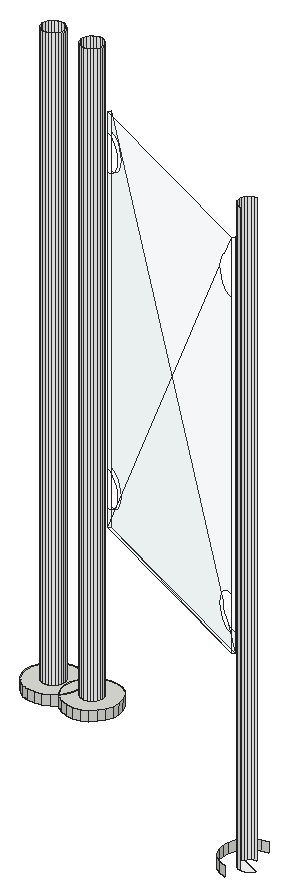
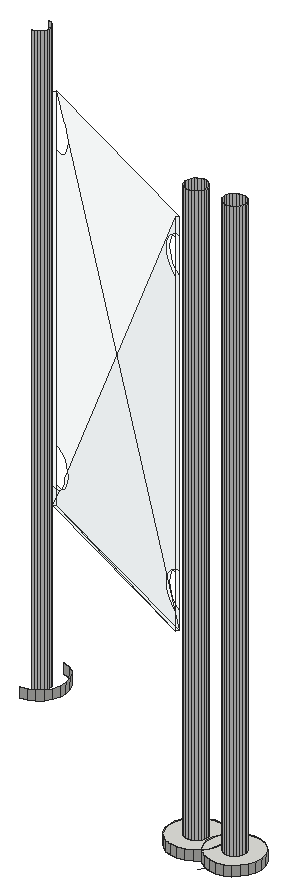
# SketchUp Ruby script. Lengths in inches.
U = 1.inch
M = Sketchup.active_model
def pt(a) = Geom::Point3d.new(a.map { |v| v * U })
def face(e, loops, mat)
  f = e.add_face(loops[0].map { |a| pt(a) })
  loops[1..].each { |l| e.add_face(l.map { |a| pt(a) }).erase! }
  f.material = f.back_material = mat if mat
  f
end
# faces: each face lists its corners as indices into pts; further lists are holes
def faces(e, pts, list, mat = nil) = list.each { |f| face(e, (f[0].is_a?(Array) ? f : [f]).map { |l| l.map { |i| pts[i] } }, mat) }
# xy, xz, yz: faces in a plane at the given z, y or x. An outline is a flat list of corners, or four numbers for a rectangle; further outlines are holes
def ring(l) = l.size == 4 ? [[l[0], l[1]], [l[2], l[1]], [l[2], l[3]], [l[0], l[3]]] : l.each_slice(2).to_a
def flat(e, list, mat, &to3) = list.each { |f| face(e, (f[0].is_a?(Array) ? f : [f]).map { |l| ring(l).map { |u, v| to3.(u, v) } }, mat) }
def xy(e, z, list, mat = nil) = flat(e, list, mat) { |x, y| [x, y, z] }
def xz(e, y, list, mat = nil) = flat(e, list, mat) { |x, z| [x, y, z] }
def yz(e, x, list, mat = nil) = flat(e, list, mat) { |y, z| [x, y, z] }
def lines(e, pts, list) = list.each { |a, b| e.add_line(pt(pts[a]), pt(pts[b])) }
# prism: a flat outline (further loops are holes) pulled along v
def prism(e, loops, v, mat = nil)
  f = face(e, loops, mat); d = Geom::Vector3d.new(v.map { |x| x * U })
  f.pushpull(f.normal.samedirection?(d) ? d.length : -d.length)
end
def box(e, o, s, mat = nil) = prism(e, [[o, [o[0] + s[0], o[1], o[2]], [o[0] + s[0], o[1] + s[1], o[2]], [o[0], o[1] + s[1], o[2]]]], [0, 0, s[2]], mat)
def at(x, y, z, deg = 0) = Geom::Transformation.translation(pt([x, y, z])) * Geom::Transformation.rotation(ORIGIN, Z_AXIS, deg.degrees)
def axes(o, x, y, z) = Geom::Transformation.new([*x, 0, *y, 0, *z, 0, *pt(o).to_a, 1])
def part(name) = M.definitions.add(name)
# library, detail: a bought-in or finely detailed component or shape, given as its bounding box
def library(name, o, s) = part(name).tap { |d| box(d.entities, o, s) }
def detail(e, o, s) = box(e.add_group.entities, o, s)
def put(e, d, t, mat = nil) = e.add_instance(d, t).tap { |i| i.material = mat if mat }
def group(e, t, mat = nil) = e.add_group.tap { |g| g.transformation = t; g.material = mat if mat }.entities
root = M.entities
M.materials.add("Glass_Safety_01").color = [204, 235, 244]
M.materials["Glass_Safety_01"].alpha = 0.1
M.materials.add("[Color_000]").color = [255, 255, 255]
xy(root,321.267,[[[557.192,657.767,557.595,657.85,557.962,658.034,558.139,658.191,558.27,658.307,558.496,658.65,558.626,659.04,558.65,659.451,558.568,659.854,558.383,660.221,558.111,660.529,557.767,660.755,557.377,660.885,556.967,660.909,556.564,660.826,556.197,660.642,555.901,660.38,555.889,660.369,555.663,660.026,555.533,659.636,555.529,659.561,555.509,659.226,555.591,658.823,555.775,658.455,555.88,658.337,556.048,658.148,556.392,657.922,556.782,657.792],[557.124,658.71,556.96,658.72,556.804,658.772,556.8,658.774,556.667,658.862,556.558,658.985,556.484,659.132,556.451,659.293,556.461,659.457,556.513,659.613,556.603,659.751,556.726,659.86,556.873,659.933,557.034,659.967,557.199,659.957,557.355,659.905,557.492,659.814,557.601,659.691,557.675,659.544,557.708,659.383,557.698,659.219,557.646,659.063,557.556,658.926,557.433,658.817,557.286,658.743]],[[554.814,657.808,555.217,657.891,555.585,658.075,555.88,658.337,555.892,658.348,556.118,658.691,556.231,659.029,556.248,659.081,556.273,659.492,556.19,659.894,556.006,660.262,555.901,660.38,555.733,660.569,555.39,660.796,555.343,660.811,555,660.925,554.589,660.95,554.186,660.867,553.819,660.683,553.511,660.41,553.285,660.067,553.155,659.677,553.131,659.266,553.214,658.864,553.398,658.496,553.671,658.189,554.014,657.962,554.404,657.833],[554.747,658.751,554.583,658.76,554.427,658.812,554.289,658.903,554.18,659.026,554.107,659.173,554.073,659.334,554.083,659.498,554.135,659.654,554.226,659.791,554.349,659.901,554.496,659.974,554.657,660.007,554.821,659.997,554.977,659.946,555.114,659.855,555.223,659.732,555.297,659.585,555.33,659.424,555.32,659.26,555.268,659.104,555.178,658.966,555.055,658.857,554.908,658.784]],[558.139,658.191,558.27,658.307,558.496,658.65,558.626,659.04,558.65,659.451,558.568,659.854,558.383,660.221,558.111,660.529,557.767,660.755,557.377,660.885,556.967,660.909,556.564,660.826,556.197,660.642,555.901,660.38,555.733,660.569,555.39,660.796,555.343,660.811,555.326,660.757,555.304,660.668,555.287,660.578,555.276,660.487,555.272,660.395,555.273,660.303,555.28,660.212,555.294,660.121,555.313,660.031,555.338,659.943,555.369,659.857,555.405,659.772,555.447,659.691,555.494,659.612,555.529,659.561,555.546,659.536,555.603,659.464,555.664,659.396,555.73,659.332,555.8,659.273,555.874,659.218,555.951,659.168,556.031,659.123,556.231,659.029,556.389,658.953,556.8,658.774,556.667,658.862,556.558,658.985,556.484,659.132,556.451,659.293,556.461,659.457,556.513,659.613,556.603,659.751,556.726,659.86,556.873,659.933,557.034,659.967,557.199,659.957,557.355,659.905,557.492,659.814,557.601,659.691,557.675,659.544,557.708,659.383,557.698,659.219,557.646,659.063,557.556,658.926,557.433,658.817,557.286,658.743,557.124,658.71,556.96,658.72,556.813,658.769]])
xy(root,321.267,[[572.658,651.259,572.819,651.292,572.966,651.366,573.089,651.475,573.18,651.612,573.188,651.637,572.038,652.138,571.995,652.006,571.985,651.842,572.018,651.681,572.092,651.534,572.201,651.411,572.338,651.321,572.494,651.269],[557.124,658.71,557.286,658.743,557.433,658.817,557.556,658.926,557.646,659.063,557.698,659.219,557.708,659.383,557.675,659.544,557.601,659.691,557.492,659.814,557.355,659.905,557.199,659.957,557.034,659.967,556.873,659.933,556.726,659.86,556.603,659.751,556.513,659.613,556.461,659.457,556.451,659.293,556.484,659.132,556.558,658.985,556.667,658.862,556.8,658.774,556.804,658.772,556.96,658.72],[554.747,658.751,554.908,658.784,555.055,658.857,555.178,658.966,555.268,659.104,555.32,659.26,555.33,659.424,555.297,659.585,555.223,659.732,555.114,659.855,554.977,659.946,554.821,659.997,554.657,660.007,554.496,659.974,554.349,659.901,554.226,659.791,554.135,659.654,554.083,659.498,554.073,659.334,554.107,659.173,554.18,659.026,554.289,658.903,554.427,658.812,554.583,658.76]],"[Color_000]")
xy(root,321.858,[[557.192,657.767,557.595,657.85,557.962,658.034,558.27,658.307,558.496,658.65,558.626,659.04,558.65,659.451,558.568,659.854,558.383,660.221,558.111,660.529,557.767,660.755,557.377,660.885,556.967,660.909,556.564,660.826,556.197,660.642,555.901,660.38,556.006,660.262,556.19,659.894,556.273,659.492,556.248,659.081,556.118,658.691,555.892,658.348,555.88,658.337,556.048,658.148,556.392,657.922,556.782,657.792],[554.814,657.808,555.217,657.891,555.585,658.075,555.88,658.337,555.775,658.455,555.591,658.823,555.509,659.226,555.533,659.636,555.663,660.026,555.889,660.369,555.901,660.38,555.733,660.569,555.39,660.796,555,660.925,554.589,660.95,554.186,660.867,553.819,660.683,553.511,660.41,553.285,660.067,553.155,659.677,553.131,659.266,553.214,658.864,553.398,658.496,553.671,658.189,554.014,657.962,554.404,657.833],[555.88,658.337,555.892,658.348,556.118,658.691,556.248,659.081,556.273,659.492,556.19,659.894,556.006,660.262,555.901,660.38,555.889,660.369,555.663,660.026,555.533,659.636,555.509,659.226,555.591,658.823,555.775,658.455]])
xy(root,331.897,[[570.999,652.552,558.812,658.398,558.897,658.576],[570.999,652.552,558.897,658.576,571.084,652.73]],"Glass_Safety_01")
p = [[571.925,650.471,321.267],[572.316,650.341,321.267],[572.316,650.341,321.858],[571.925,650.471,321.858],[571.582,650.697,321.267],[571.582,650.697,321.858],
  [571.309,651.004,321.267],[571.309,651.004,321.858],[571.125,651.372,321.267],[571.125,651.372,321.858],[572.201,651.411,321.267],[572.338,651.321,321.267],
  [572.338,651.321,357.267],[572.201,651.411,357.267],[572.494,651.269,321.267],[572.494,651.269,357.267],[571.043,651.775,321.267],[571.043,651.775,321.858],
  [572.092,651.534,321.267],[572.092,651.534,357.267],[572.018,651.681,321.267],[572.018,651.681,357.267],[571.985,651.842,321.267],[571.985,651.842,357.267],
  [571.067,652.185,321.267],[571.067,652.185,321.858],[571.995,652.006,321.267],[571.995,652.006,357.267],[572.047,652.162,321.267],[572.038,652.138,321.267],
  [572.047,652.162,357.267],[571.197,652.575,321.267],[571.176,652.513,321.267],[571.197,652.575,321.858],[572.137,652.3,321.267],[572.137,652.3,357.267],
  [572.26,652.409,321.267],[572.26,652.409,357.267],[572.407,652.482,321.267],[572.407,652.482,357.267],[572.568,652.515,321.267],[572.568,652.515,357.267],
  [571.423,652.918,321.267],[571.423,652.918,321.858],[571.73,653.191,321.267],[571.73,653.191,321.858],[572.098,653.375,321.267],[572.098,653.375,321.858],
  [572.501,653.458,321.267],[572.501,653.458,321.858],[554.014,657.962,321.267],[554.404,657.833,321.267],[554.404,657.833,321.858],[554.014,657.962,321.858],
  [554.814,657.808,321.267],[554.814,657.808,321.858],[555.217,657.891,321.267],[555.217,657.891,321.858],[556.392,657.922,321.267],[556.782,657.792,321.267],
  [556.782,657.792,321.858],[556.392,657.922,321.858],[557.192,657.767,321.267],[557.192,657.767,321.858],[557.595,657.85,321.267],[557.595,657.85,321.858],
  [555.585,658.075,321.267],[555.585,658.075,321.858],[556.048,658.148,321.267],[556.048,658.148,321.858],[557.962,658.034,321.267],[557.962,658.034,321.858],
  [553.671,658.189,321.267],[553.671,658.189,321.858],[558.139,658.191,321.267],[558.27,658.307,321.267],[558.27,658.307,321.858],[555.88,658.337,321.267],
  [555.892,658.348,321.267],[555.892,658.348,321.858],[555.88,658.337,321.858],[555.775,658.455,321.267],[555.775,658.455,321.858],[553.398,658.496,321.267],
  [553.398,658.496,321.858],[556.118,658.691,321.267],[556.118,658.691,321.858],[558.496,658.65,321.267],[558.496,658.65,321.858],[553.214,658.864,321.267],
  [553.214,658.864,321.858],[555.591,658.823,321.267],[555.591,658.823,321.858],[556.231,659.029,321.267],[556.248,659.081,321.267],[556.248,659.081,321.858],
  [556.804,658.772,321.267],[556.813,658.769,321.267],[556.96,658.72,321.267],[556.96,658.72,357.267],[556.804,658.772,357.267],[557.124,658.71,321.267],
  [557.124,658.71,357.267],[557.286,658.743,321.267],[557.286,658.743,357.267],[557.433,658.817,321.267],[557.433,658.817,357.267],[558.626,659.04,321.267],
  [558.626,659.04,321.858],[554.289,658.903,321.267],[554.427,658.812,321.267],[554.427,658.812,357.267],[554.289,658.903,357.267],[554.583,658.76,321.267],
  [554.583,658.76,357.267],[554.747,658.751,321.267],[554.747,658.751,357.267],[554.908,658.784,321.267],[554.908,658.784,357.267],[555.055,658.857,321.267],
  [555.055,658.857,357.267],[555.509,659.226,321.267],[555.509,659.226,321.858],[556.667,658.862,321.267],[556.8,658.774,321.267],[556.667,658.862,357.267],
  [557.556,658.926,321.267],[557.556,658.926,357.267],[553.131,659.266,321.267],[553.131,659.266,321.858],[554.18,659.026,321.267],[554.18,659.026,357.267],
  [555.178,658.966,321.267],[555.178,658.966,357.267],[556.558,658.985,321.267],[556.558,658.985,357.267],[557.646,659.063,321.267],[557.646,659.063,357.267],
  [554.107,659.173,321.267],[554.107,659.173,357.267],[555.268,659.104,321.267],[555.268,659.104,357.267],[556.484,659.132,321.267],[556.484,659.132,357.267],
  [558.65,659.451,321.267],[558.65,659.451,321.858],[555.32,659.26,321.267],[555.32,659.26,357.267],[556.273,659.492,321.267],[556.273,659.492,321.858],
  [556.451,659.293,321.267],[556.451,659.293,357.267],[557.698,659.219,321.267],[557.698,659.219,357.267],[554.073,659.334,321.267],[554.073,659.334,357.267],
  [555.533,659.636,321.267],[555.529,659.561,321.267],[555.533,659.636,321.858],[557.708,659.383,321.267],[557.708,659.383,357.267],[553.155,659.677,321.267],
  [553.155,659.677,321.858],[554.083,659.498,321.267],[554.083,659.498,357.267],[555.33,659.424,321.267],[555.33,659.424,357.267],[556.461,659.457,321.267],
  [556.461,659.457,357.267],[555.297,659.585,321.267],[555.297,659.585,357.267],[557.675,659.544,321.267],[557.675,659.544,357.267],[554.135,659.654,321.267],
  [554.135,659.654,357.267],[556.19,659.894,321.267],[556.19,659.894,321.858],[556.513,659.613,321.267],[556.513,659.613,357.267],[557.601,659.691,321.267],
  [557.601,659.691,357.267],[558.568,659.854,321.267],[558.568,659.854,321.858],[555.223,659.732,321.267],[555.223,659.732,357.267],[555.663,660.026,321.267],
  [555.663,660.026,321.858],[556.603,659.751,321.267],[556.603,659.751,357.267],[553.285,660.067,321.267],[553.285,660.067,321.858],[554.226,659.791,321.267],
  [554.226,659.791,357.267],[555.114,659.855,321.267],[555.114,659.855,357.267],[557.492,659.814,321.267],[557.492,659.814,357.267],[554.349,659.901,321.267],
  [554.349,659.901,357.267],[556.726,659.86,321.267],[556.726,659.86,357.267],[557.355,659.905,321.267],[557.355,659.905,357.267],[554.496,659.974,321.267],
  [554.496,659.974,357.267],[554.977,659.946,321.267],[554.821,659.997,321.267],[554.821,659.997,357.267],[554.977,659.946,357.267],[556.006,660.262,321.267],
  [556.006,660.262,321.858],[556.873,659.933,321.267],[556.873,659.933,357.267],[557.034,659.967,321.267],[557.034,659.967,357.267],[557.199,659.957,321.267],
  [557.199,659.957,357.267],[558.383,660.221,321.267],[558.383,660.221,321.858],[554.657,660.007,321.267],[554.657,660.007,357.267],[555.889,660.369,321.267],
  [555.889,660.369,321.858],[553.511,660.41,321.267],[553.511,660.41,321.858],[558.111,660.529,321.267],[558.111,660.529,321.858],[555.901,660.38,321.267],
  [555.733,660.569,321.267],[555.733,660.569,321.858],[555.901,660.38,321.858],[553.819,660.683,321.267],[553.819,660.683,321.858],[556.197,660.642,321.267],
  [556.197,660.642,321.858],[557.767,660.755,321.267],[557.767,660.755,321.858],[555.39,660.796,321.267],[555.39,660.796,321.858],[556.564,660.826,321.267],
  [556.564,660.826,321.858],[554.186,660.867,321.267],[554.186,660.867,321.858],[555.343,660.811,321.267],[555,660.925,321.267],[555,660.925,321.858],
  [556.967,660.909,321.267],[556.967,660.909,321.858],[557.377,660.885,321.267],[557.377,660.885,321.858],[554.589,660.95,321.267],[554.589,660.95,321.858],
  [558.812,658.398,351.283],[558.812,658.398,335.126],[559.06,658.279,335.089],[559.291,658.168,334.983],[559.489,658.073,334.814],[559.642,658,334.594],
  [559.738,657.954,334.338],[559.77,657.938,334.0625],[559.738,657.954,333.787],[559.642,658,333.531],[559.489,658.073,333.311],[559.291,658.168,333.142],
  [559.06,658.279,333.036],[558.812,658.398,333],[558.812,658.398,331.897],[569.839,653.109,352.36],[569.87,653.094,352.621],[569.966,653.048,352.877],
  [570.118,652.975,353.098],[570.317,652.88,353.267],[570.332,652.873,353.273],[570.999,652.552,354.511],[558.812,658.398,354.511],[558.812,658.398,353.409],
  [559.06,658.279,353.373],[559.291,658.168,353.267],[559.489,658.073,353.098],[559.642,658,352.877],[559.738,657.954,352.621],[559.77,657.938,352.346],
  [559.738,657.954,352.071],[559.642,658,351.815],[559.489,658.073,351.594],[559.291,658.168,351.425],[559.06,658.279,351.319],[570.999,652.552,335.126],
  [570.999,652.552,351.283],[570.796,652.65,351.283],[570.548,652.769,351.319],[570.317,652.88,351.425],[570.118,652.975,351.594],[569.966,653.048,351.815],
  [569.87,653.094,352.071],[569.837,653.11,352.346],[570.999,652.552,331.897],[570.999,652.552,333],[570.796,652.65,333],[570.548,652.769,333.036],
  [570.317,652.88,333.142],[570.118,652.975,333.311],[569.966,653.048,333.531],[569.87,653.094,333.787],[569.837,653.11,334.0625],[569.87,653.094,334.338],
  [569.966,653.048,334.594],[570.118,652.975,334.814],[570.317,652.88,334.983],[570.548,652.769,335.089],[570.796,652.65,335.126],[571.084,652.73,331.897],
  [571.084,652.73,333],[571.084,652.73,335.126],[571.084,652.73,351.283],[571.084,652.73,353.409],[571.084,652.73,354.511],[570.999,652.552,353.409],
  [558.897,658.576,331.897],[558.897,658.576,333],[559.145,658.457,333.036],[559.376,658.346,333.142],[559.575,658.251,333.311],[559.727,658.178,333.531],
  [559.823,658.132,333.787],[559.855,658.116,334.0625],[559.823,658.132,334.338],[559.727,658.178,334.594],[559.575,658.251,334.814],[559.376,658.346,334.983],
  [559.145,658.457,335.089],[558.897,658.576,335.126],[558.897,658.576,351.283],[559.145,658.457,351.319],[559.376,658.346,351.425],[559.575,658.251,351.594],
  [559.727,658.178,351.815],[559.823,658.132,352.071],[559.855,658.116,352.346],[559.823,658.132,352.621],[559.727,658.178,352.877],[559.575,658.251,353.098],
  [559.376,658.346,353.267],[559.145,658.457,353.373],[558.897,658.576,353.409],[558.897,658.576,354.511],[569.924,653.286,334.049],[569.955,653.271,333.787],
  [570.051,653.225,333.531],[570.203,653.152,333.311],[570.402,653.057,333.142],[570.417,653.05,333.135],[570.633,652.946,333.036],[570.881,652.827,333],
  [555.5,661.213,321.267],[555.354,660.844,321.267]]
faces(root,p,[[0,1,2,3],[4,0,3,5],[6,4,5,7],[8,6,7,9],[16,8,9,17],[24,16,17,25],[31,32,24,25,33],[42,31,33,43],
  [44,42,43,45],[46,44,45,47],[48,46,47,49],[50,51,52,53],[51,54,55,52],[54,56,57,55],[58,59,60,61],[59,62,63,60],
  [62,64,65,63],[56,66,67,57],[68,58,61,69],[64,70,71,65],[72,50,53,73],[70,74,75,76,71],[66,77,78,79,80,67],[81,77,68,69,80,82],
  [83,72,73,84],[78,85,86,79],[75,87,88,76],[89,83,84,90],[91,81,82,92],[85,93,94,95,86],[87,107,108,88],[121,91,92,122],
  [128,89,90,129],[107,144,145,108],[94,148,149,95],[156,157,121,122,158],[161,128,129,162],[148,175,176,149],[144,181,182,145],[185,156,158,186],
  [189,161,162,190],[175,209,210,176],[181,217,218,182],[221,185,186,222],[223,189,190,224],[217,225,226,218],[209,227,228,229,230,210],[231,223,224,232],
  [233,227,221,222,230,234],[225,235,236,226],[228,237,238,229],[239,233,234,240],[241,231,232,242],[237,243,244,245,238],[246,239,240,247],[235,248,249,236],
  [250,241,242,251],[244,250,251,245],[248,246,247,249]])
faces(root,p,[[10,11,12,13],[11,14,15,12],[18,10,13,19],[20,18,19,21],[22,20,21,23],[26,22,23,27],[28,29,26,27,30],[34,28,30,35],
  [36,34,35,37],[38,36,37,39],[40,38,39,41],[96,97,98,99,100],[98,101,102,99],[101,103,104,102],[103,105,106,104],[109,110,111,112],
  [110,113,114,111],[113,115,116,114],[115,117,118,116],[117,119,120,118],[123,124,96,100,125],[105,126,127,106],[130,109,112,131],[119,132,133,120],
  [134,123,125,135],[126,136,137,127],[138,130,131,139],[132,140,141,133],[142,134,135,143],[140,146,147,141],[150,142,143,151],[136,152,153,137],
  [154,138,139,155],[152,159,160,153],[163,154,155,164],[146,165,166,147],[167,150,151,168],[165,169,170,166],[159,171,172,160],[173,163,164,174],
  [177,167,168,178],[171,179,180,172],[169,183,184,170],[187,177,178,188],[191,173,174,192],[183,193,194,184],[179,195,196,180],[197,191,192,198],
  [199,187,188,200],[195,201,202,196],[203,197,198,204],[205,206,207,208],[193,205,208,194],[211,199,200,212],[213,211,212,214],[201,215,216,202],
  [219,203,204,220],[206,219,220,207],[215,213,214,216]],"[Color_000]")
faces(root,p,[[252,253,254,255,256,257,258,259,260,261,262,263,264,265,266,267,268,269,270,271,272,273,274,275,276,277,278,279,280,281,282,283,284,285,286],[287,288,289,290,291,292,293,294,295,267,266,296,297,298,299,300,301,302,303,304,305,306,307,308,309,310],[296,311,312,313,314,315,316,273,317,288,287,297],[318,319,320,321,322,323,324,325,326,327,328,329,330,331,332,333,334,335,336,337,338,339,340,341,342,343,344,345,346,347,348,349,350,351,311],[311,351,352,353,312],[318,266,265,253,252,275,274,345,344,332,331,319]],"Glass_Safety_01")
lines(root,p,[[354,355],[355,243]])
